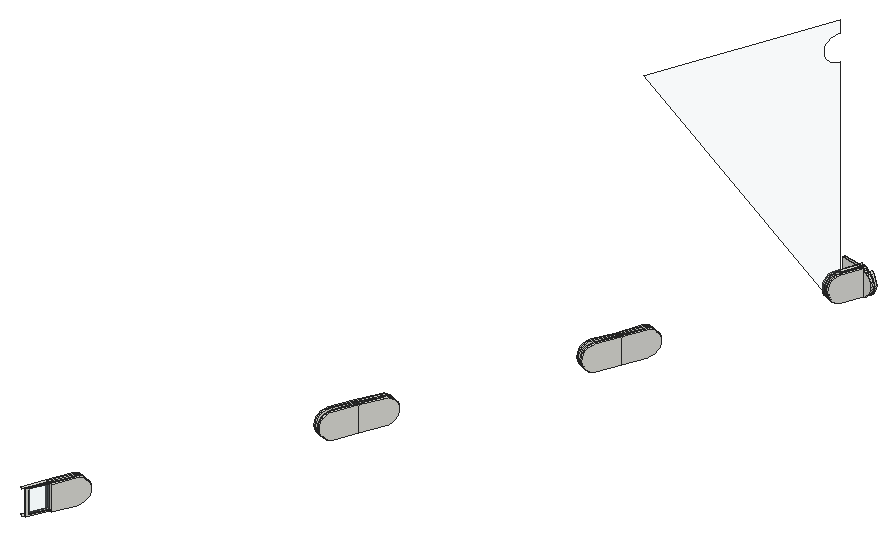
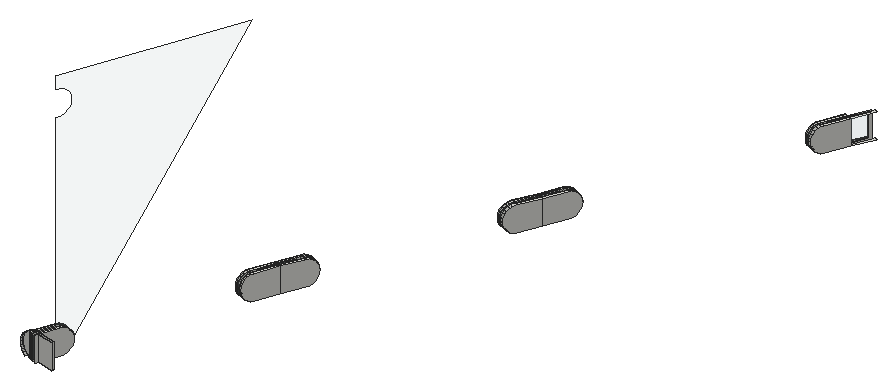
# SketchUp Ruby script. Lengths in inches.
U = 1.inch
M = Sketchup.active_model
def pt(a) = Geom::Point3d.new(a.map { |v| v * U })
def face(e, loops, mat)
  f = e.add_face(loops[0].map { |a| pt(a) })
  loops[1..].each { |l| e.add_face(l.map { |a| pt(a) }).erase! }
  f.material = f.back_material = mat if mat
  f
end
# faces: each face lists its corners as indices into pts; further lists are holes
def faces(e, pts, list, mat = nil) = list.each { |f| face(e, (f[0].is_a?(Array) ? f : [f]).map { |l| l.map { |i| pts[i] } }, mat) }
# xy, xz, yz: faces in a plane at the given z, y or x. An outline is a flat list of corners, or four numbers for a rectangle; further outlines are holes
def ring(l) = l.size == 4 ? [[l[0], l[1]], [l[2], l[1]], [l[2], l[3]], [l[0], l[3]]] : l.each_slice(2).to_a
def flat(e, list, mat, &to3) = list.each { |f| face(e, (f[0].is_a?(Array) ? f : [f]).map { |l| ring(l).map { |u, v| to3.(u, v) } }, mat) }
def xy(e, z, list, mat = nil) = flat(e, list, mat) { |x, y| [x, y, z] }
def xz(e, y, list, mat = nil) = flat(e, list, mat) { |x, z| [x, y, z] }
def yz(e, x, list, mat = nil) = flat(e, list, mat) { |y, z| [x, y, z] }
def lines(e, pts, list) = list.each { |a, b| e.add_line(pt(pts[a]), pt(pts[b])) }
# prism: a flat outline (further loops are holes) pulled along v
def prism(e, loops, v, mat = nil)
  f = face(e, loops, mat); d = Geom::Vector3d.new(v.map { |x| x * U })
  f.pushpull(f.normal.samedirection?(d) ? d.length : -d.length)
end
def box(e, o, s, mat = nil) = prism(e, [[o, [o[0] + s[0], o[1], o[2]], [o[0] + s[0], o[1] + s[1], o[2]], [o[0], o[1] + s[1], o[2]]]], [0, 0, s[2]], mat)
def at(x, y, z, deg = 0) = Geom::Transformation.translation(pt([x, y, z])) * Geom::Transformation.rotation(ORIGIN, Z_AXIS, deg.degrees)
def axes(o, x, y, z) = Geom::Transformation.new([*x, 0, *y, 0, *z, 0, *pt(o).to_a, 1])
def part(name) = M.definitions.add(name)
# library, detail: a bought-in or finely detailed component or shape, given as its bounding box
def library(name, o, s) = part(name).tap { |d| box(d.entities, o, s) }
def detail(e, o, s) = box(e.add_group.entities, o, s)
def put(e, d, t, mat = nil) = e.add_instance(d, t).tap { |i| i.material = mat if mat }
def group(e, t, mat = nil) = e.add_group.tap { |g| g.transformation = t; g.material = mat if mat }.entities
root = M.entities
M.materials.add("Glass_Safety_01").color = [204, 235, 244]
M.materials["Glass_Safety_01"].alpha = 0.1
xy(root,333,[[998.772,953.408,998.52,953.518,999.306,955.322,999.558,955.212,998.837,953.555],[999.992,955.024,999.739,955.134,1000.525,956.939,1000.778,956.828],[999.558,955.212,999.306,955.322,1000.092,957.127,1000.344,957.017],[1008.551,974.677,1008.298,974.787,1008.365,974.939,1009.084,976.592,1009.337,976.482],[1008.118,974.865,1007.865,974.976,1008.651,976.78,1008.904,976.67,1008.184,975.017],
  [1009.337,976.482,1009.084,976.592,1009.871,978.396,1010.123,978.286],[1008.904,976.67,1008.651,976.78,1009.4375,978.585,1009.69,978.475],[1016.523,992.981,1016.271,993.091,1016.348,993.269,1017.057,994.896,1017.309,994.786],[1016.09,993.17,1015.837,993.28,1016.618,995.072,1016.875,994.971,1016.168,993.348],[1017.315,994.799,1017.058,994.9,1017.774,996.733,1018.031,996.633],
  [1016.875,994.971,1016.618,995.072,1016.621,995.078,1016.624,995.085,1016.876,994.975],[1016.876,994.975,1016.624,995.085,1017.334,996.905,1017.591,996.805],[1023.511,1010.674,1023.255,1010.774,1023.329,1010.964,1023.838,1012.27,1023.906,1012.255,1023.948,1012.447,1023.965,1012.524,1023.982,1012.603,1024.227,1012.508],[1023.071,1010.846,1022.815,1010.946,1023.371,1012.372,1023.644,1012.3125,1023.145,1011.036],[1023.906,1012.255,1023.838,1012.27,1023.911,1012.456,1023.948,1012.447],
  [1023.838,1012.27,1023.799,1012.279,1023.841,1012.471,1023.911,1012.456],[1023.799,1012.279,1023.644,1012.3125,1023.716,1012.498,1023.841,1012.471],[1023.644,1012.3125,1023.371,1012.372,1023.444,1012.558,1023.716,1012.498],[1023.948,1012.447,1023.911,1012.456,1023.94,1012.53,1023.965,1012.524],[1023.911,1012.456,1023.841,1012.471,1023.858,1012.548,1023.94,1012.53],
  [1023.841,1012.471,1023.716,1012.498,1023.745,1012.572,1023.858,1012.548]])
xy(root,333.078,[[999.11,953.69,998.93,953.769,999.558,955.212,999.739,955.134],[999.739,955.134,999.558,955.212,1000.187,956.656,1000.368,956.578],[1008.456,975.148,1008.275,975.226,1008.904,976.67,1009.084,976.592],[1009.084,976.592,1008.904,976.67,1009.533,978.114,1009.713,978.035],[1016.428,993.452,1016.247,993.531,1016.875,994.971,1016.966,994.936,1017.057,994.896],
  [1017.058,994.9,1016.966,994.936,1016.876,994.975,1017.447,996.438,1017.631,996.367],[1016.966,994.936,1016.875,994.971,1016.875,994.973,1016.876,994.975],[1023.398,1011.141,1023.214,1011.213,1023.745,1012.572,1023.858,1012.548,1023.879,1012.644,1023.97,1012.608]],"Glass_Safety_01")
xy(root,335.047,[[999.11,953.69,999.739,955.134,999.558,955.212,998.93,953.769],[999.739,955.134,1000.368,956.578,1000.187,956.656,999.558,955.212],[1008.456,975.148,1009.084,976.592,1008.904,976.67,1008.275,975.226],[1009.084,976.592,1009.713,978.035,1009.533,978.114,1008.904,976.67],[1016.428,993.452,1017.057,994.896,1016.966,994.936,1016.875,994.971,1016.247,993.531],
  [1017.058,994.9,1017.631,996.367,1017.447,996.438,1016.876,994.975,1016.966,994.936],[1016.966,994.936,1016.876,994.975,1016.875,994.973,1016.875,994.971],[1023.398,1011.141,1023.97,1012.608,1023.879,1012.644,1023.858,1012.548,1023.745,1012.572,1023.214,1011.213]],"Glass_Safety_01")
xy(root,335.125,[[998.772,953.408,998.837,953.555,999.558,955.212,999.306,955.322,998.52,953.518],[999.992,955.024,1000.778,956.828,1000.525,956.939,999.739,955.134],[999.558,955.212,1000.344,957.017,1000.092,957.127,999.306,955.322],[1008.551,974.677,1009.337,976.482,1009.084,976.592,1008.365,974.939,1008.298,974.787],[1008.118,974.865,1008.184,975.017,1008.904,976.67,1008.651,976.78,1007.865,974.976],
  [1009.337,976.482,1010.123,978.286,1009.871,978.396,1009.084,976.592],[1008.904,976.67,1009.69,978.475,1009.4375,978.585,1008.651,976.78],[1016.523,992.981,1017.309,994.786,1017.057,994.896,1016.348,993.269,1016.271,993.091],[1016.09,993.17,1016.168,993.348,1016.875,994.971,1016.618,995.072,1015.837,993.28],[1017.315,994.799,1018.031,996.633,1017.774,996.733,1017.058,994.9],
  [1016.875,994.971,1016.876,994.975,1016.624,995.085,1016.621,995.078,1016.618,995.072],[1016.876,994.975,1017.591,996.805,1017.334,996.905,1016.624,995.085],[1023.511,1010.674,1024.227,1012.508,1023.982,1012.603,1023.965,1012.524,1023.948,1012.447,1023.906,1012.255,1023.838,1012.27,1023.329,1010.964,1023.255,1010.774],[1023.071,1010.846,1023.145,1011.036,1023.644,1012.3125,1023.371,1012.372,1022.815,1010.946],[1023.906,1012.255,1023.948,1012.447,1023.911,1012.456,1023.838,1012.27],
  [1023.838,1012.27,1023.911,1012.456,1023.841,1012.471,1023.799,1012.279],[1023.799,1012.279,1023.841,1012.471,1023.716,1012.498,1023.644,1012.3125],[1023.644,1012.3125,1023.716,1012.498,1023.444,1012.558,1023.371,1012.372],[1023.948,1012.447,1023.965,1012.524,1023.94,1012.53,1023.911,1012.456],[1023.911,1012.456,1023.94,1012.53,1023.858,1012.548,1023.841,1012.471],
  [1023.841,1012.471,1023.858,1012.548,1023.745,1012.572,1023.716,1012.498]])
p = [[999.739,955.134,333],[999.017,953.477,333],[999.017,953.477,335.125],[999.739,955.134,335.125],[999.739,955.134,335.047],[999.11,953.69,335.047],
  [999.11,953.69,333.078],[999.739,955.134,333.078],[999.558,955.212,335.125],[998.837,953.555,335.125],[998.837,953.555,333],[999.558,955.212,333],
  [999.558,955.212,333.078],[998.93,953.769,333.078],[998.93,953.769,335.047],[999.558,955.212,335.047],[999.992,955.024,335.125],[999.992,955.024,333],
  [1000.778,956.828,335.125],[1000.778,956.828,333],[1000.887,957.081,333.036],[1000.99,957.316,333.142],[1001.078,957.518,333.311],[1001.145,957.672,333.531],
  [1001.1875,957.77,333.787],[1001.202,957.803,334.0625],[1001.1875,957.77,334.338],[1001.145,957.672,334.594],[1001.078,957.518,334.814],[1000.99,957.316,334.983],
  [1000.887,957.081,335.089],[1000.525,956.939,335.125],[1000.525,956.939,333],[1000.368,956.578,333.078],[1000.368,956.578,335.047],[999.306,955.322,333],
  [999.306,955.322,335.125],[1000.344,957.017,333],[1000.344,957.017,335.125],[1000.187,956.656,335.047],[1000.187,956.656,333.078],[1000.092,957.127,335.125],
  [1000.202,957.379,335.089],[1000.304,957.614,334.983],[1000.392,957.816,334.814],[1000.459,957.971,334.594],[1000.502,958.069,334.338],[1000.516,958.102,334.0625],
  [1000.502,958.069,333.787],[1000.459,957.971,333.531],[1000.392,957.816,333.311],[1000.304,957.614,333.142],[1000.202,957.379,333.036],[1000.092,957.127,333],
  [1000.635,957.191,333.036],[1000.737,957.426,333.142],[1000.825,957.628,333.311],[1000.893,957.783,333.531],[1000.935,957.88,333.787],[1000.949,957.913,334.0625],
  [1000.935,957.88,334.338],[1000.893,957.783,334.594],[1000.825,957.628,334.814],[1000.737,957.426,334.983],[1000.635,957.191,335.089],[1000.454,957.269,333.036],
  [1000.454,957.269,335.089],[1000.557,957.504,334.983],[1000.645,957.706,334.814],[1000.712,957.861,334.594],[1000.754,957.958,334.338],[1000.769,957.992,334.0625],
  [1000.754,957.958,333.787],[1000.712,957.861,333.531],[1000.645,957.706,333.311],[1000.557,957.504,333.142],[1009.337,976.482,335.125],[1008.551,974.677,335.125],
  [1008.441,974.425,335.089],[1008.339,974.19,334.983],[1008.251,973.988,334.814],[1008.184,973.833,334.594],[1008.141,973.735,334.338],[1008.127,973.702,334.0625],
  [1008.141,973.735,333.787],[1008.184,973.833,333.531],[1008.251,973.988,333.311],[1008.339,974.19,333.142],[1008.441,974.425,333.036],[1008.551,974.677,333],
  [1009.337,976.482,333],[1008.298,974.787,335.125],[1008.365,974.939,335.125],[1008.365,974.939,333],[1008.298,974.787,333],[1008.189,974.535,333.036],
  [1008.086,974.3,333.142],[1007.998,974.098,333.311],[1007.931,973.943,333.531],[1007.888,973.846,333.787],[1007.874,973.8125,334.0625],[1007.888,973.846,334.338],
  [1007.931,973.943,334.594],[1007.998,974.098,334.814],[1008.086,974.3,334.983],[1008.189,974.535,335.089],[1008.118,974.865,333],[1008.184,975.017,333],
  [1008.184,975.017,335.125],[1008.118,974.865,335.125],[1008.008,974.613,335.089],[1007.906,974.378,334.983],[1007.818,974.176,334.814],[1007.75,974.021,334.594],
  [1007.708,973.924,334.338],[1007.694,973.891,334.0625],[1007.708,973.924,333.787],[1007.75,974.021,333.531],[1007.818,974.176,333.311],[1007.906,974.378,333.142],
  [1008.008,974.613,333.036],[1007.865,974.976,335.125],[1008.651,976.78,335.125],[1008.651,976.78,333],[1007.865,974.976,333],[1007.755,974.723,333.036],
  [1007.653,974.488,333.142],[1007.565,974.286,333.311],[1007.498,974.132,333.531],[1007.455,974.034,333.787],[1007.441,974.001,334.0625],[1007.455,974.034,334.338],
  [1007.498,974.132,334.594],[1007.565,974.286,334.814],[1007.653,974.488,334.983],[1007.755,974.723,335.089],[1009.084,976.592,333],[1009.084,976.592,335.125],
  [1009.084,976.592,335.047],[1008.456,975.148,335.047],[1008.456,975.148,333.078],[1009.084,976.592,333.078],[1008.904,976.67,335.125],[1008.904,976.67,333],
  [1008.904,976.67,333.078],[1008.275,975.226,333.078],[1008.275,975.226,335.047],[1008.904,976.67,335.047],[1010.123,978.286,335.125],[1010.123,978.286,333],
  [1010.233,978.539,333.036],[1010.335,978.774,333.142],[1010.423,978.975,333.311],[1010.491,979.13,333.531],[1010.533,979.228,333.787],[1010.548,979.261,334.0625],
  [1010.533,979.228,334.338],[1010.491,979.13,334.594],[1010.423,978.975,334.814],[1010.335,978.774,334.983],[1010.233,978.539,335.089],[1009.871,978.396,335.125],
  [1009.871,978.396,333],[1009.713,978.035,333.078],[1009.713,978.035,335.047],[1009.69,978.475,333],[1009.69,978.475,335.125],[1009.533,978.114,335.047],
  [1009.533,978.114,333.078],[1009.4375,978.585,335.125],[1009.547,978.837,335.089],[1009.65,979.072,334.983],[1009.737,979.274,334.814],[1009.805,979.429,334.594],
  [1009.847,979.526,334.338],[1009.862,979.56,334.0625],[1009.847,979.526,333.787],[1009.805,979.429,333.531],[1009.737,979.274,333.311],[1009.65,979.072,333.142],
  [1009.547,978.837,333.036],[1009.4375,978.585,333],[1009.98,978.649,333.036],[1010.083,978.884,333.142],[1010.171,979.086,333.311],[1010.238,979.24,333.531],
  [1010.28,979.338,333.787],[1010.295,979.371,334.0625],[1010.28,979.338,334.338],[1010.238,979.24,334.594],[1010.171,979.086,334.814],[1010.083,978.884,334.983],
  [1009.98,978.649,335.089],[1009.8,978.727,333.036],[1009.8,978.727,335.089],[1009.902,978.962,334.983],[1009.99,979.164,334.814],[1010.058,979.319,334.594],
  [1010.1,979.416,334.338],[1010.114,979.45,334.0625],[1010.1,979.416,333.787],[1010.058,979.319,333.531],[1009.99,979.164,333.311],[1009.902,978.962,333.142],
  [1017.309,994.786,335.125],[1016.523,992.981,335.125],[1016.413,992.729,335.089],[1016.311,992.494,334.983],[1016.223,992.292,334.814],[1016.156,992.137,334.594],
  [1016.113,992.04,334.338],[1016.099,992.007,334.0625],[1016.113,992.04,333.787],[1016.156,992.137,333.531],[1016.223,992.292,333.311],[1016.311,992.494,333.142],
  [1016.413,992.729,333.036],[1016.523,992.981,333],[1017.309,994.786,333],[1016.271,993.091,335.125],[1016.348,993.269,335.125],[1016.348,993.269,333],
  [1016.271,993.091,333],[1016.161,992.839,333.036],[1016.058,992.604,333.142],[1015.97,992.402,333.311],[1015.903,992.247,333.531],[1015.861,992.15,333.787],
  [1015.846,992.117,334.0625],[1015.861,992.15,334.338],[1015.903,992.247,334.594],[1015.97,992.402,334.814],[1016.058,992.604,334.983],[1016.161,992.839,335.089],
  [1016.09,993.17,333],[1016.168,993.348,333],[1016.875,994.971,333],[1016.875,994.971,333.078],[1016.875,994.971,335.047],[1016.875,994.971,335.125],
  [1016.168,993.348,335.125],[1016.09,993.17,335.125],[1015.98,992.918,335.089],[1015.878,992.683,334.983],[1015.79,992.481,334.814],[1015.723,992.326,334.594],
  [1015.68,992.229,334.338],[1015.666,992.195,334.0625],[1015.68,992.229,333.787],[1015.723,992.326,333.531],[1015.79,992.481,333.311],[1015.878,992.683,333.142],
  [1015.98,992.918,333.036],[1015.837,993.28,335.125],[1016.618,995.072,335.125],[1016.618,995.072,333],[1015.837,993.28,333],[1015.728,993.028,333.036],
  [1015.625,992.793,333.142],[1015.537,992.591,333.311],[1015.47,992.436,333.531],[1015.427,992.339,333.787],[1015.413,992.306,334.0625],[1015.427,992.339,334.338],
  [1015.47,992.436,334.594],[1015.537,992.591,334.814],[1015.625,992.793,334.983],[1015.728,993.028,335.089],[1017.057,994.896,333],[1017.057,994.896,335.125],
  [1017.057,994.896,335.047],[1016.428,993.452,335.047],[1016.428,993.452,333.078],[1017.057,994.896,333.078],[1017.058,994.9,333.078],[1017.058,994.9,333],
  [1017.315,994.799,333],[1017.315,994.799,335.125],[1017.058,994.9,335.125],[1017.058,994.9,335.047],[1018.031,996.633,335.125],[1018.031,996.633,333],
  [1018.131,996.89,333.036],[1018.224,997.128,333.142],[1018.304,997.333,333.311],[1018.365,997.491,333.531],[1018.404,997.59,333.787],[1018.417,997.623,334.0625],
  [1018.404,997.59,334.338],[1018.365,997.491,334.594],[1018.304,997.333,334.814],[1018.224,997.128,334.983],[1018.131,996.89,335.089],[1017.774,996.733,335.125],
  [1017.774,996.733,333],[1017.631,996.367,333.078],[1017.631,996.367,335.047],[1016.876,994.975,333.078],[1016.876,994.975,333],[1016.624,995.085,333],
  [1016.624,995.085,335.125],[1016.876,994.975,335.125],[1016.876,994.975,335.047],[1017.591,996.805,333],[1017.691,997.061,333.036],[1017.784,997.3,333.142],
  [1017.864,997.505,333.311],[1017.925,997.663,333.531],[1017.964,997.762,333.787],[1017.977,997.795,334.0625],[1017.964,997.762,334.338],[1017.925,997.663,334.594],
  [1017.864,997.505,334.814],[1017.784,997.3,334.983],[1017.691,997.061,335.089],[1017.591,996.805,335.125],[1016.621,995.078,333],[1016.621,995.078,335.125],
  [1017.334,996.905,335.125],[1017.434,997.162,335.089],[1017.527,997.4,334.983],[1017.607,997.605,334.814],[1017.669,997.763,334.594],[1017.707,997.862,334.338],
  [1017.72,997.895,334.0625],[1017.707,997.862,333.787],[1017.669,997.763,333.531],[1017.607,997.605,333.311],[1017.527,997.4,333.142],[1017.434,997.162,333.036],
  [1017.334,996.905,333],[1017.874,996.99,333.036],[1017.967,997.229,333.142],[1018.047,997.434,333.311],[1018.109,997.591,333.531],[1018.147,997.69,333.787],
  [1018.16,997.724,334.0625],[1018.147,997.69,334.338],[1018.109,997.591,334.594],[1018.047,997.434,334.814],[1017.967,997.229,334.983],[1017.874,996.99,335.089],
  [1024.227,1012.508,335.125],[1023.511,1010.674,335.125],[1023.411,1010.418,335.089],[1023.318,1010.179,334.983],[1023.238,1009.974,334.814],[1023.177,1009.817,334.594],
  [1023.138,1009.718,334.338],[1023.125,1009.684,334.0625],[1023.138,1009.718,333.787],[1023.177,1009.817,333.531],[1023.238,1009.974,333.311],[1023.318,1010.179,333.142],
  [1023.411,1010.418,333.036],[1023.511,1010.674,333],[1024.227,1012.508,333],[1023.255,1010.774,335.125],[1023.329,1010.964,335.125],[1023.329,1010.964,333],
  [1023.255,1010.774,333],[1023.155,1010.518,333.036],[1023.061,1010.279,333.142],[1022.981,1010.074,333.311],[1022.92,1009.917,333.531],[1022.881,1009.818,333.787],
  [1022.868,1009.784,334.0625],[1022.881,1009.818,334.338],[1022.92,1009.917,334.594],[1022.981,1010.074,334.814],[1023.061,1010.279,334.983],[1023.155,1010.518,335.089],
  [1022.725,1009.958,333.61],[1022.798,1010.146,333.311],[1022.798,1010.147,333.31],[1022.878,1010.351,333.142],[1022.971,1010.59,333.036],[1023.071,1010.846,333],
  [1023.145,1011.036,333],[1023.145,1011.036,335.125],[1023.071,1010.846,335.125],[1022.971,1010.59,335.089],[1022.878,1010.351,334.983],[1022.798,1010.146,334.814],
  [1022.737,1009.988,334.594],[1022.698,1009.889,334.338],[1022.685,1009.856,334.0625],[1022.698,1009.889,333.787],[1023.473,1012.632,335.125],[1023.53,1012.78,335.125],
  [1023.53,1012.78,333],[1023.473,1012.632,333],[1023.444,1012.558,333],[1023.371,1012.372,333],[1022.815,1010.946,333],[1022.715,1010.69,333.036],
  [1022.621,1010.451,333.142],[1022.541,1010.246,333.311],[1022.48,1010.089,333.531],[1022.441,1009.99,333.787],[1022.428,1009.956,334.0625],[1022.441,1009.99,334.338],
  [1022.48,1010.089,334.594],[1022.541,1010.246,334.814],[1022.621,1010.451,334.983],[1022.715,1010.69,335.089],[1022.815,1010.946,335.125],[1023.371,1012.372,335.125],
  [1023.444,1012.558,335.125],[1023.644,1012.3125,335.125],[1023.644,1012.3125,333],[1023.716,1012.498,333],[1023.745,1012.572,333],[1023.787,1012.68,333],
  [1023.787,1012.68,333.078],[1023.745,1012.572,333.078],[1023.214,1011.213,333.078],[1023.214,1011.213,335.047],[1023.745,1012.572,335.047],[1023.787,1012.68,335.047],
  [1023.787,1012.68,335.125],[1023.745,1012.572,335.125],[1023.716,1012.498,335.125],[1023.838,1012.27,333],[1023.838,1012.27,335.125],[1023.911,1012.456,335.125],
  [1023.94,1012.53,335.125],[1023.97,1012.608,335.125],[1023.97,1012.608,335.047],[1023.398,1011.141,335.047],[1023.398,1011.141,333.078],[1023.97,1012.608,333.078],
  [1023.97,1012.608,333],[1023.94,1012.53,333],[1023.911,1012.456,333],[1023.799,1012.279,335.125],[1023.799,1012.279,333],[1023.906,1012.255,333],
  [1024.175,1012.196,333.036],[1024.425,1012.142,333.142],[1024.641,1012.095,333.311],[1024.806,1012.059,333.531],[1024.909,1012.036,333.787],[1024.945,1012.028,334.0625],
  [1024.909,1012.036,334.338],[1024.806,1012.059,334.594],[1024.641,1012.095,334.814],[1024.425,1012.142,334.983],[1024.175,1012.196,335.089],[1023.906,1012.255,335.125],
  [1024.217,1012.389,333.036],[1024.467,1012.334,333.142],[1023.251,1012.599,335.125],[1022.025,1012.868,335.125],[1022.025,1012.868,333],[1023.251,1012.599,333],
  [1023.841,1012.471,333],[1023.948,1012.447,333],[1024.683,1012.287,333.311],[1024.848,1012.251,333.531],[1024.951,1012.228,333.787],[1024.987,1012.22,334.0625],
  [1024.951,1012.228,334.338],[1024.848,1012.251,334.594],[1024.683,1012.287,334.814],[1024.467,1012.334,334.983],[1024.217,1012.389,335.089],[1023.948,1012.447,335.125],
  [1023.841,1012.471,335.125],[1021.983,1012.675,335.125],[1021.983,1012.675,333],[1023.858,1012.548,333],[1023.858,1012.548,333.078],[1023.858,1012.548,335.047],
  [1023.858,1012.548,335.125],[1023.965,1012.524,335.125],[1024.234,1012.466,335.089],[1024.484,1012.411,334.983],[1024.699,1012.364,334.814],[1024.864,1012.328,334.594],
  [1024.968,1012.305,334.338],[1025.003,1012.297,334.0625],[1024.968,1012.305,333.787],[1024.864,1012.328,333.531],[1024.699,1012.364,333.311],[1024.484,1012.411,333.142],
  [1024.234,1012.466,333.036],[1023.965,1012.524,333],[1016.247,993.531,335.047],[1016.247,993.531,333.078],[1016.966,994.936,333.078],[1016.966,994.936,335.047],
  [1016.875,994.973,335.047],[1016.875,994.973,333.078],[1017.447,996.438,333.078],[1017.447,996.438,335.047],[1024.526,1012.603,333.142],[1024.741,1012.556,333.311],
  [1022.737,1009.988,333.531],[1024.906,1012.52,333.531],[1025.01,1012.497,333.787],[1023.145,1011.036,351.283],[1017.591,996.805,354.511],[1023.145,1011.036,354.511],
  [1023.145,1011.036,353.409],[1023.071,1010.846,353.409],[1022.971,1010.59,353.373],[1022.878,1010.351,353.267],[1022.798,1010.146,353.098],[1022.737,1009.988,352.877],
  [1022.698,1009.889,352.621],[1022.685,1009.856,352.346],[1022.698,1009.889,352.071],[1022.737,1009.988,351.814],[1022.798,1010.146,351.594],[1022.878,1010.351,351.425],
  [1022.971,1010.59,351.319],[1023.071,1010.846,351.283],[1025.046,1012.49,334.0625],[1025.01,1012.497,334.338],[1024.906,1012.52,334.594],[1024.741,1012.556,334.814],
  [1024.526,1012.603,334.983]]
faces(root,p,[[0,1,2,3,4,5,6,7],[8,9,10,11,12,13,14,15],[0,7,4,3,16,17],[18,16,17,19,20,21,22,23,24,25,26,27,28,29,30],[3,31,32,0,7,33,34,4],[12,11,35,36,8,15],[11,37,38,8,15,39,40,12],[36,41,42,43,44,45,46,47,48,49,50,51,52,53,35],
  [32,54,20,19],[65,37,53,52],[54,55,21,20],[75,65,52,51],[76,77,78,79,80,81,82,83,84,85,86,87,88,89,90],[91,92,93,94,95,96,97,98,99,100,101,102,103,104,105],[106,107,108,109,110,111,112,113,114,115,116,117,118,119,120],[121,122,123,124,125,126,127,128,129,130,131,132,133,134,135],
  [96,95,88,87],[120,119,126,125],[95,94,89,88],[106,120,125,124],[136,93,92,137,138,139,140,141],[142,108,107,143,144,145,146,147],[136,141,138,137,76,90],[148,76,90,149,150,151,152,153,154,155,156,157,158,159,160],
  [137,161,162,136,141,163,164,138],[144,143,123,122,142,147],[143,165,166,142,147,167,168,144],[122,169,170,171,172,173,174,175,176,177,178,179,180,181,123],[162,182,150,149],[193,165,181,180],[182,183,151,150],[203,193,180,179],
  [204,205,206,207,208,209,210,211,212,213,214,215,216,217,218],[219,220,221,222,223,224,225,226,227,228,229,230,231,232,233],[234,235,236,237,238,239,240,241,242,243,244,245,246,247,248,249,250,251,252],[253,254,255,256,257,258,259,260,261,262,263,264,265,266,267],[224,223,216,215],[252,251,258,257],[223,222,217,216],[234,252,257,256],
  [268,221,220,269,270,271,272,273],[268,273,270,269,204,218],[274,275,276,277,278,279],[280,277,276,281,282,283,284,285,286,287,288,289,290,291,292],[278,293,294,275,274,295,296,279],[236,237,238,239,254,255],[297,298,299,300,301,302],[301,239,238,237,236,298,297,302],
  [301,239,238,237,236,298,303,304,305,306,307,308,309,310,311,312,313,314,315],[316,255,254,317,300,299],[254,317,300,318,319,320,321,322,323,324,325,326,327,328,329,330,299,316,255],[294,331,282,281],[304,303,330,329],[331,332,283,282],[305,304,329,328],[342,343,344,345,346,347,348,349,350,351,352,353,354,355,356],
  [357,358,359,360,361,362,363,364,365,366,367,368,369,370,371],[388,389,390,391,392,393,394,395,396,397,398,399,400,401,402,403,404,405,406,407,408],[362,361,354,353],[376,375,396,395],[361,360,355,354],[377,376,395,394],[409,379,378,410,411,412,413,414,415,416,417,418,419,420,421,422],[423,359,358,424,425,426,427,428,429,430,431,432,433,434],
  [424,435,436,423,437,438,439,440,441,442,443,444,445,446,447,448,449],[438,450,451,439],[452,453,454,455,392,411,456,434,457,450,451,458,459,460,461,462,463,464,465,466,467,425,468,422,408],[437,457,450,438],[410,436,435,409,407,469,470,393],[471,472,473,474,468,435,436,456],[433,471,472,473,474,426,475,476,477,478,479,480,481,482,483,484,485,486,487],[485,451,450,486],
  [486,450,457,487],[55,56,22,21],[74,75,51,50],[97,96,87,86],[119,118,127,126],[183,184,152,151],[202,203,179,178],[225,224,215,214],
  [251,250,259,258],[332,333,284,283],[306,305,328,327],[363,362,353,352],[374,373,397,396,375],[439,451,458,440],[484,458,451,485],[496,497,484,485],
  [56,57,23,22],[73,74,50,49],[98,97,86,85],[118,117,128,127],[184,185,153,152],[201,202,178,177],[226,225,214,213],[250,249,260,259],
  [333,334,285,284],[307,306,327,326],[364,363,352,351],[373,498,398,397],[372,498,373],[440,458,459,441],[483,459,458,484],[497,499,483,484],
  [57,58,24,23],[72,73,49,48],[99,98,85,84],[117,116,129,128],[185,186,154,153],[200,201,177,176],[227,226,213,212],[249,248,261,260],
  [334,335,286,285],[308,307,326,325],[365,364,351,350],[372,387,399,398,498],[441,459,460,442],[482,460,459,483],[499,500,482,483],[58,59,25,24],
  [71,72,48,47],[100,99,84,83],[116,115,130,129],[186,187,155,154],[199,200,176,175],[228,227,212,211],[248,247,262,261],[335,336,287,286],
  [309,308,325,324],[366,365,350,349],[387,386,400,399],[442,460,461,443],[481,461,460,482],[500,518,481,482],[59,60,26,25],[70,71,47,46],
  [101,100,83,82],[115,114,131,130],[187,188,156,155],[198,199,175,174],[229,228,211,210],[247,246,263,262],[336,337,288,287],[310,309,324,323],
  [367,366,349,348],[386,385,401,400],[443,461,462,444],[480,462,461,481],[518,519,480,481],[60,61,27,26],[69,70,46,45],[102,101,82,81],
  [114,113,132,131],[188,189,157,156],[197,198,174,173],[230,229,210,209],[246,245,264,263],[337,338,289,288],[311,310,323,322],[368,367,348,347],
  [385,384,402,401],[444,462,463,445],[479,463,462,480],[519,520,479,480],[61,62,28,27],[68,69,45,44],[103,102,81,80],[113,112,133,132],
  [189,190,158,157],[196,197,173,172],[231,230,209,208],[245,244,265,264],[338,339,290,289],[312,311,322,321],[369,368,347,346],[384,383,403,402],
  [445,463,464,446],[478,464,463,479],[520,521,478,479],[62,63,29,28],[67,68,44,43],[104,103,80,79],[112,111,134,133],[190,191,159,158],
  [195,196,172,171],[232,231,208,207],[244,243,266,265],[339,340,291,290],[313,312,321,320],[370,369,346,345],[383,382,404,403],[446,464,465,447],
  [477,465,464,478],[521,522,477,478],[63,64,30,29],[66,67,43,42],[105,104,79,78],[111,110,135,134],[191,192,160,159],[194,195,171,170],
  [233,232,207,206],[243,242,267,266],[340,341,292,291],[314,313,320,319],[371,370,345,344],[382,381,405,404],[447,465,466,448],[476,466,465,477],
  [64,31,18,30],[38,66,42,41],[91,105,78,77],[110,109,121,135],[192,161,148,160],[166,194,170,169],[219,233,206,205],[242,241,253,267],
  [341,293,280,292],[315,314,319,318],[357,371,344,343],[381,380,406,405],[466,448,449,467]])
faces(root,p,[[31,32,54,55,56,57,58,59,60,61,62,63,64],[37,38,66,67,68,69,70,71,72,73,74,75,65],[161,162,182,183,184,185,186,187,188,189,190,191,192],[165,166,194,195,196,197,198,199,200,201,202,203,193],[293,294,331,332,333,334,335,336,337,338,339,340,341],[303,315,314,313,312,311,310,309,308,307,306,305,304],[372,373,374,375,376,377,378,379,380,381,382,383,384,385,386,387],[7,6,5,4],
  [13,12,15,14],[15,4,7,12],[33,7,4,34],[12,40,39,15],[34,33,40,39],[140,139,146,145],[141,140,139,138],[145,144,147,146],
  [147,138,141,144],[163,141,138,164],[144,168,167,147],[164,163,168,167],[272,271,488,489],[488,238,237,489],[273,272,271,270],[490,491,238,237],
  [302,491,490,297],[273,490,491,270],[491,490,274,279],[295,274,279,296],[492,302,297,493,237,238],[494,297,302,495],[295,494,495,296],[430,429,417,416],
  [431,430,429,428],[415,414,419,418,417,416],[501,379,380,381,382,383,384,385,386,387,372,502,503,504,505,506,507,508,509,510,511,512,513,514,515,516,517]],"Glass_Safety_01")
